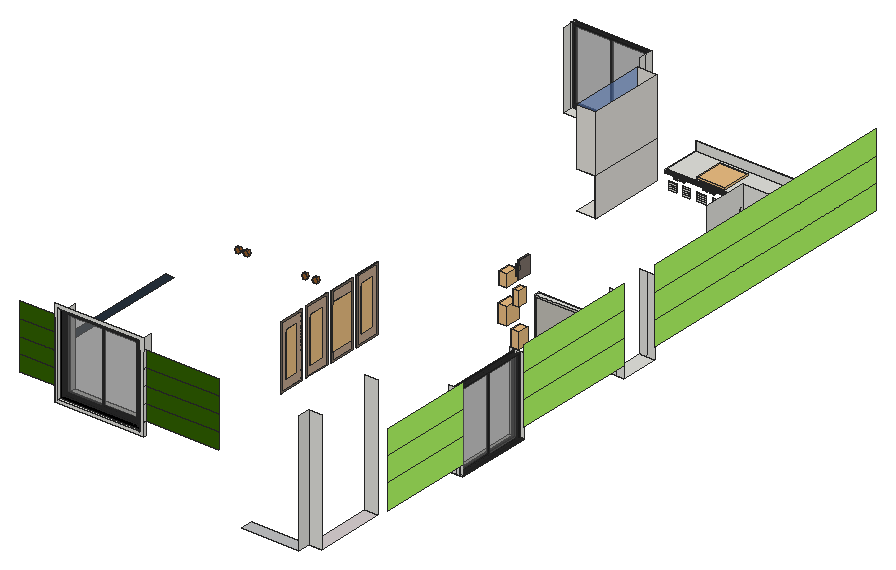
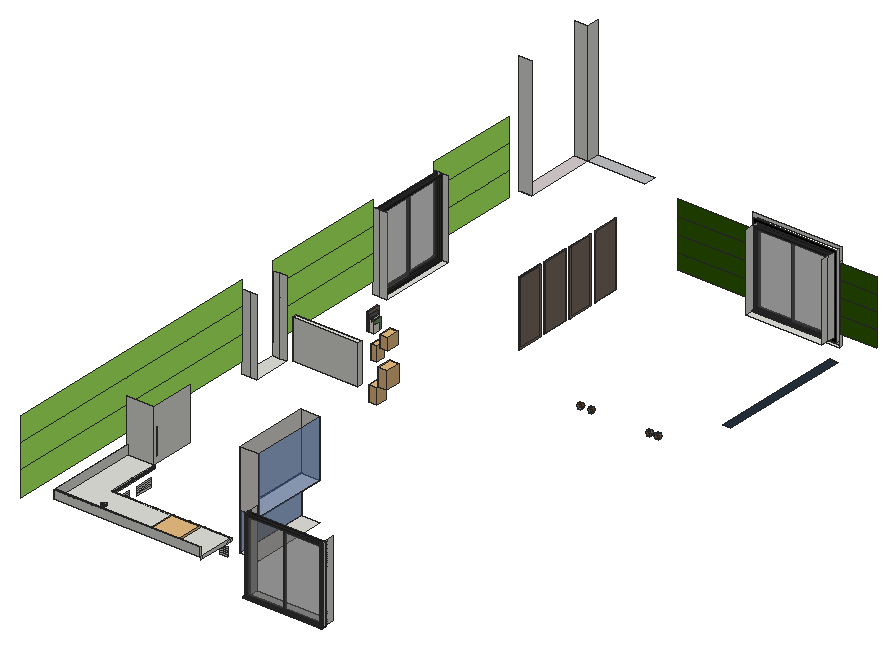
# SketchUp Ruby script. Lengths in inches.
U = 1.inch
M = Sketchup.active_model
def pt(a) = Geom::Point3d.new(a.map { |v| v * U })
def face(e, loops, mat)
  f = e.add_face(loops[0].map { |a| pt(a) })
  loops[1..].each { |l| e.add_face(l.map { |a| pt(a) }).erase! }
  f.material = f.back_material = mat if mat
  f
end
# faces: each face lists its corners as indices into pts; further lists are holes
def faces(e, pts, list, mat = nil) = list.each { |f| face(e, (f[0].is_a?(Array) ? f : [f]).map { |l| l.map { |i| pts[i] } }, mat) }
# xy, xz, yz: faces in a plane at the given z, y or x. An outline is a flat list of corners, or four numbers for a rectangle; further outlines are holes
def ring(l) = l.size == 4 ? [[l[0], l[1]], [l[2], l[1]], [l[2], l[3]], [l[0], l[3]]] : l.each_slice(2).to_a
def flat(e, list, mat, &to3) = list.each { |f| face(e, (f[0].is_a?(Array) ? f : [f]).map { |l| ring(l).map { |u, v| to3.(u, v) } }, mat) }
def xy(e, z, list, mat = nil) = flat(e, list, mat) { |x, y| [x, y, z] }
def xz(e, y, list, mat = nil) = flat(e, list, mat) { |x, z| [x, y, z] }
def yz(e, x, list, mat = nil) = flat(e, list, mat) { |y, z| [x, y, z] }
def lines(e, pts, list) = list.each { |a, b| e.add_line(pt(pts[a]), pt(pts[b])) }
# prism: a flat outline (further loops are holes) pulled along v
def prism(e, loops, v, mat = nil)
  f = face(e, loops, mat); d = Geom::Vector3d.new(v.map { |x| x * U })
  f.pushpull(f.normal.samedirection?(d) ? d.length : -d.length)
end
def box(e, o, s, mat = nil) = prism(e, [[o, [o[0] + s[0], o[1], o[2]], [o[0] + s[0], o[1] + s[1], o[2]], [o[0], o[1] + s[1], o[2]]]], [0, 0, s[2]], mat)
def at(x, y, z, deg = 0) = Geom::Transformation.translation(pt([x, y, z])) * Geom::Transformation.rotation(ORIGIN, Z_AXIS, deg.degrees)
def axes(o, x, y, z) = Geom::Transformation.new([*x, 0, *y, 0, *z, 0, *pt(o).to_a, 1])
def part(name) = M.definitions.add(name)
# library, detail: a bought-in or finely detailed component or shape, given as its bounding box
def library(name, o, s) = part(name).tap { |d| box(d.entities, o, s) }
def detail(e, o, s) = box(e.add_group.entities, o, s)
def put(e, d, t, mat = nil) = e.add_instance(d, t).tap { |i| i.material = mat if mat }
def group(e, t, mat = nil) = e.add_group.tap { |g| g.transformation = t; g.material = mat if mat }.entities
root = M.entities
M.materials.add("[0127_Magenta]").color = [213, 211, 206]
M.materials.add("[0136_Charcoal]").color = [35, 35, 35]
M.materials.add("[1A2796_Cherry-on-Top]1").color = [40, 37, 35]
M.materials.add("[1D2827_Elegant-Rose]").color = [193, 166, 142]
M.materials.add("[1P0222_Buff-Apricot]").color = [122, 108, 96]
M.materials.add("[Color F01]").color = [47, 96, 0]
M.materials.add("[Color F03]").color = [178, 255, 101]
M.materials.add("[Color M09]").color = [0, 0, 0]
M.materials.add("[Color M09]2").color = [194, 192, 183]
M.materials.add("[Color_006]").color = [86, 86, 86]
M.materials.add("[Concrete Pavers Block Multi]").color = [124, 140, 145]
M.materials.add("[Fencing Metal Straight]").color = [194, 195, 196]
M.materials.add("[Fencing Railing Metal]").color = [216, 207, 208]
M.materials.add("[Marble Carrara Gold Floor Tile]").color = [225, 223, 217]
M.materials.add("[Translucent Glass Blue]").color = [100, 149, 237]
M.materials["[Translucent Glass Blue]"].alpha = 0.5
M.materials.add("[Translucent Glass Gray]").color = [117, 117, 117]
M.materials["[Translucent Glass Gray]"].alpha = 0.39
M.materials.add("[Translucent_Glass_Gray]").color = [128, 128, 128]
M.materials["[Translucent_Glass_Gray]"].alpha = 0.5
M.materials.add("[Wood Floor Parquet]").color = [145, 89, 39]
M.materials.add("ksiazki_bialy").color = [255, 246, 235]
M.materials.add("ksiazki_bok").color = [126, 114, 106]
M.materials.add("ksiazki_color").color = [116, 147, 106]
M.materials.add("ksiazki_front").color = [107, 97, 79]
M.materials.add("ksiazki_kolor").color = [96, 96, 96]
M.materials.add("wire_1").color = [39, 49, 60]
c1 = library("Figurine display case",[0,0,0],[10.24,10.24,12.53])
c2 = part("Window")
box(c2.entities,[0,0,0],[39.75,0.5,77],"[Translucent Glass Gray]")
c3 = part("Slider2")
put(c3.entities,c2,at(1.25,1,1.25),"[Translucent Glass Gray]")
c4 = part("Slider")
prism(c4.entities,[[[0,0,0],[42.25,0,0],[42.25,0,79.5],[0,0,79.5]],[[41,0,1.25],[1.25,0,1.25],[1.25,0,78.25],[41,0,78.25]]],[0,1.5,0],"[0136_Charcoal]")
put(c4.entities,c2,at(1.25,1,1.25),"[Translucent_Glass_Gray]")
c5 = part("Frame\#1")
xy(c5.entities,0,[[0,0,88,0.25],[0,6.25,88,6.5]],"[0136_Charcoal]")
xy(c5.entities,1.25,[[-1,6.25,0,9.5],[88,6.25,89,9.5],[0,6.5,88,9.5]],"[0136_Charcoal]")
xy(c5.entities,2,[[2,0.25,86,6.25]],"[0136_Charcoal]")
xy(c5.entities,2.25,[[2.25,0,85.75,1.25],[2.25,2,85.75,5],[2.25,5.75,85.75,6.5],[88,6.25,89,6.25,88,6.5]],"[0136_Charcoal]")
xy(c5.entities,2.75,[[2.75,1.25,85.25,2],[2.75,5,85.25,5.75]],"[0136_Charcoal]")
xy(c5.entities,81.25,[[2.75,1.25,85.25,2],[2.75,5,85.25,5.75]],"[0136_Charcoal]")
xy(c5.entities,81.75,[[2.25,0,85.75,1.25],[2.25,2,85.75,5],[2.25,5.75,85.75,6.5]],"[0136_Charcoal]")
xy(c5.entities,82,[[2,0.25,86,6.25]],"[0136_Charcoal]")
xy(c5.entities,84,[[0,0,88,0.25],[0,6.25,88,6.5]],"[0136_Charcoal]")
xz(c5.entities,0,[[[0,0,88,84],[2.25,2.25,85.75,81.75]]],"[0136_Charcoal]")
xz(c5.entities,0.25,[[[0,0,88,84],[2,2,86,82]]],"[0136_Charcoal]")
xz(c5.entities,1.25,[[[2.25,2.25,85.75,81.75],[2.75,2.75,85.25,81.25]]],"[0136_Charcoal]")
xz(c5.entities,2,[[[2.25,2.25,85.75,81.75],[2.75,2.75,85.25,81.25]]],"[0136_Charcoal]")
xz(c5.entities,5,[[[2.25,2.25,85.75,81.75],[2.75,2.75,85.25,81.25]]],"[0136_Charcoal]")
xz(c5.entities,5.75,[[[2.25,2.25,85.75,81.75],[2.75,2.75,85.25,81.25]]],"[0136_Charcoal]")
xz(c5.entities,6.25,[[[0,0,88,0,88,1.25,89,1.25,89,2.25,88,2.25,88,84,0,84,0,2.25,-1,2.25,-1,1.25,0,1.25],[2,2,86,82]]],"[0136_Charcoal]")
xz(c5.entities,6.5,[[0,0,88,1.25],[0,2.25,0,84,88,84,88,2.25,85.75,2.25,85.75,81.75,2.25,81.75,2.25,2.25]],"[0136_Charcoal]")
xz(c5.entities,9.5,[[-1,1.25,89,1.75]],"[0136_Charcoal]")
yz(c5.entities,-1,[[6.25,1.25,6.25,2.25,9.5,1.75,9.5,1.25]],"[0136_Charcoal]")
yz(c5.entities,0,[[0,0,0.25,84],[6.25,0,6.5,1.25],[6.25,2.25,6.5,84]],"[0136_Charcoal]")
yz(c5.entities,2,[[0.25,2,6.25,82]],"[0136_Charcoal]")
yz(c5.entities,2.25,[[0,2.25,1.25,81.75],[2,2.25,5,81.75],[5.75,2.25,6.5,81.75]],"[0136_Charcoal]")
yz(c5.entities,2.75,[[1.25,2.75,2,81.25],[5,2.75,5.75,81.25]],"[0136_Charcoal]")
yz(c5.entities,85.25,[[1.25,2.75,2,81.25],[5,2.75,5.75,81.25]],"[0136_Charcoal]")
yz(c5.entities,85.75,[[0,2.25,1.25,81.75],[2,2.25,5,81.75],[5.75,2.25,6.5,81.75]],"[0136_Charcoal]")
yz(c5.entities,86,[[0.25,2,6.25,82]],"[0136_Charcoal]")
yz(c5.entities,88,[[0,0,0.25,84],[6.25,0,6.5,1.25],[6.25,2.25,6.5,84]],"[0136_Charcoal]")
yz(c5.entities,89,[[6.25,1.25,9.5,1.25,9.5,1.75,6.25,2.25]],"[0136_Charcoal]")
p = [[89,6.25,2.25],[89,9.5,1.75],[88,6.5,2.25],[-1,6.25,2.25],[0,6.25,2.25],[-1,9.5,1.75],
  [0,6.5,2.25],[2.25,6.5,2.25],[85.75,6.5,2.25]]
faces(c5.entities,p,[[0,1,2],[3,4,5],[6,5,4],[6,7,8,2,1,5]],"[0136_Charcoal]")
put(c5.entities,c3,axes([1.48,-2.48,1.48],[1.01887,0,0],[0,5.47515,0],[0,0,1.01974]))
put(c5.entities,c4,at(43.5,3.5,2.25),"[Color_006]")
c6 = part("Sliding glass door")
put(c6.entities,c5,at(-89,-9.5,-1.25),"[Color_006]")
c7 = library("Range_Countertop\#1",[0,-0.11,0],[27,21.23,1.125])
c8 = library("Figurine display case \#1",[0,0,0],[10.24,10.24,12.53])
c9 = part("faucet_quarter")
xy(c9.entities,0,[[0,0,0,0.97,0.26,0.97,0.71,0.71,0.97,0.26,0.97,0]])
xy(c9.entities,4.5,[[0,0,0.71,0,0.71,0.19,0.52,0.52,0.19,0.71,0,0.71]])
xz(c9.entities,0.97,[[0,0,0.26,4.375]])
yz(c9.entities,0.97,[[0,0,0.26,4.375]])
p = [[0.71,0.71,0],[0.71,0.71,4.375],[0.97,0.26,4.375],[0.97,0.26,0],[0.26,0.97,0],[0.26,0.97,4.375],
  [0.71,0.19,4.5],[0.71,0,4.5],[0.97,0,4.375],[0.52,0.52,4.5],[0.19,0.71,4.5],[0,0.97,4.375],
  [0,0.71,4.5]]
faces(c9.entities,p,[[0,1,2,3],[4,5,1,0],[6,7,8,2],[2,1,9,6],[5,10,9,1],[5,11,12,10]])
c10 = part("Water_Faucet_Sink_Modern")
prism(c10.entities,[[[1.22,-0.07,0.65],[1.02,0.11,0.74],[1.22,0.29,0.83],[1.42,0.11,0.74]]],[0,-0.43,0.9])
xy(c10.entities,2.61,[[-0.12,-2.86,0.11,-0.36]])
xy(c10.entities,3.48,[[-0.11,-3.31,0.12,-0.36]])
xz(c10.entities,-3.31,[[-0.43,3.14,0.44,3.14,0.4375,3.16,0.32,3.36,0.12,3.48,-0.11,3.48,-0.32,3.37,-0.43,3.17]])
xz(c10.entities,-1,[[-0.1875,0.75,0.1875,2.25]])
p = [[-0.01,-3.05,2.56],[0.25,-3.15,2.68],[0.24,-3.34,2.91],[-0.02,-3.43,3.02],[-0.28,-3.33,2.89],[-0.27,-3.14,2.66],
  [-0.12,-2.86,2.61],[0.11,-2.86,2.61],[0.32,-2.96,2.73],[0.43,-3.125,2.93],[0.44,-3.31,3.14],[-0.43,-3.31,3.14],
  [-0.4375,-3.13,2.93],[-0.32,-2.96,2.73],[0.25,-3.01,2.79],[-0.01,-2.91,2.67],[-0.27,-3,2.78],[-0.28,-3.2,3.01],
  [-0.02,-3.3,3.13],[0.24,-3.21,3.02],[-0.12,-0.36,2.61],[-0.32,-0.36,2.73],[0.32,-0.36,2.73],[0.11,-0.36,2.61],
  [-0.4375,-0.36,2.93],[0.43,-0.36,2.93],[-0.43,-3.31,3.17],[-0.43,-0.36,3.17],[0.4375,-3.31,3.16],[0.4375,-0.36,3.16],
  [-0.32,-3.31,3.37],[-0.32,-0.36,3.37],[0.32,-3.31,3.36],[0.32,-0.36,3.36],[-0.11,-3.31,3.48],[-0.11,-0.36,3.48],
  [0.12,-3.31,3.48],[0.12,-0.36,3.48]]
faces(c10.entities,p,[[0,1,2,3,4,5],[[6,7,8,9,10,11,12,13],[14,15,16,17,18,19]],[15,14,1,0],[16,15,0,5],[20,6,13,21],[22,8,7,23],[17,16,5,4],[14,19,2,1],
  [21,13,12,24],[25,9,8,22],[18,17,4,3],[19,18,3,2],[24,12,11,26,27],[28,10,9,25,29],[26,30,31,27],[32,28,29,33],
  [30,34,35,31],[36,32,33,37]])
put(c10.entities,c9,at(0,0,0))
put(c10.entities,c9,at(0,0,0,90))
put(c10.entities,c9,at(0,0,0,180))
put(c10.entities,c9,at(0,0,0,-90))
c11 = part("Group\#8")
xy(c11.entities,0,[[[-2.25,-2.38,53.86,142.58],[0,0,51.61,140.2]],[0,0,51.61,140.2]])
xy(c11.entities,0.7,[[[-2.25,-2.38,53.86,142.58],[0,0,51.61,140.2]]])
xy(c11.entities,0.7,[[0,0,51.61,140.2]],"[1D2827_Elegant-Rose]")
xy(c11.entities,1.41,[[[-2.25,-2.38,53.86,142.58],[0,0,51.61,140.2]]],"[1P0222_Buff-Apricot]")
xz(c11.entities,-2.38,[[-2.25,0,53.86,0.7],[-2.25,0.7,53.86,1.41]])
xz(c11.entities,0,[[0,0,51.61,0.7],[0,0.7,51.61,1.41]])
xz(c11.entities,140.2,[[0,0,51.61,0.7],[0,0.7,51.61,1.41]])
xz(c11.entities,142.58,[[-2.25,0,53.86,0.7],[-2.25,0.7,53.86,1.41]])
yz(c11.entities,-2.25,[[-2.38,0,142.58,0.7],[-2.38,0.7,142.58,1.41]])
yz(c11.entities,0,[[0,0,140.2,0.7],[0,0.7,140.2,1.41]])
yz(c11.entities,51.61,[[0,0,140.2,0.7],[0,0.7,140.2,1.41]])
yz(c11.entities,53.86,[[-2.38,0,142.58,0.7],[-2.38,0.7,142.58,1.41]])
c12 = library("Group\#17",[0,0,0],[49.77,99.98,0.7])
c13 = library("Groupe\#36",[0,0,0],[8.85,8.01,13.18])
c14 = library("Group\#7",[0,0,0],[32.82,100.33,0.7])
c15 = library("Group\#10",[0,0,0],[29.16,100.07,0.7])
c16 = library("Group\#6",[0,0,0],[27.2,98.94,0.7])
c17 = library("vase3mm",[-1.8,-1.8,0],[3.6,3.6,4.77])
c18 = part("books")
g1 = group(c18.entities,at(0,-187.6875,-13.27))
xy(g1,13.89,[[0,1.25,0,67.05,71.57,67.05,71.57,5.87,43.27,5.87,43.27,1.25],[0,68.28,98.43,86.07]],"ksiazki_front")
xy(g1,69.43,[[0,0,43.27,5.87]],"ksiazki_bialy")
xy(g1,89.27,[[0,21.18,71.57,31.42]],"ksiazki_bialy")
xy(g1,90.86,[[0,5.87,71.57,19.73]],"ksiazki_bialy")
xy(g1,91.92,[[0,19.73,71.57,21.18]],"ksiazki_bialy")
xy(g1,101.14,[[0,31.42,71.57,40.16]],"ksiazki_bialy")
xy(g1,105.94,[[0,40.16,71.57,48.94]],"ksiazki_bialy")
xy(g1,124.42,[[0,57.01,71.57,67.05]],"ksiazki_bialy")
xy(g1,127.59,[[0,48.94,71.57,57.01]],"ksiazki_bialy")
xz(g1,5.87,[[43.27,13.89,71.57,13.89,71.57,90.86,0,90.86,0,69.43,43.27,69.43]],"ksiazki_color")
xz(g1,19.73,[[0,90.86,71.57,91.92]],"ksiazki_front")
xz(g1,21.18,[[0,89.27,71.57,91.92]],"ksiazki_front")
xz(g1,31.42,[[0,89.27,71.57,101.14]],"ksiazki_bialy")
xz(g1,40.16,[[0,101.14,71.57,105.94]],"ksiazki_color")
xz(g1,48.94,[[0,105.94,71.57,127.59]],"ksiazki_kolor")
xz(g1,57.01,[[0,124.42,71.57,127.59]],"ksiazki_front")
xz(g1,67.05,[[0,13.89,71.57,124.42]],"ksiazki_front")
yz(g1,0,[[1.25,13.89,0,69.43,5.87,69.43,5.87,90.86,19.73,90.86,19.73,91.92,21.18,91.92,21.18,89.27,31.42,89.27,31.42,101.14,40.16,101.14,40.16,105.94,48.94,105.94,48.94,127.59,57.01,127.59,57.01,124.42,67.05,124.42,67.05,13.89],[68.28,13.89,69.91,143.31,89.63,141.875,86.07,13.89]],"ksiazki_bialy")
yz(g1,43.27,[[1.25,13.89,5.87,13.89,5.87,69.43,0,69.43]],"ksiazki_front")
yz(g1,71.57,[[5.87,13.89,67.05,13.89,67.05,124.42,57.01,124.42,57.01,127.59,48.94,127.59,48.94,105.94,40.16,105.94,40.16,101.14,31.42,101.14,31.42,89.27,21.18,89.27,21.18,91.92,19.73,91.92,19.73,90.86,5.87,90.86]],"ksiazki_front")
yz(g1,98.43,[[68.28,13.89,86.07,13.89,89.63,141.875,69.91,143.31]],"ksiazki_front")
p = [[0,0,69.43],[0,1.25,13.89],[43.27,1.25,13.89],[43.27,0,69.43],[98.43,68.28,13.89],[98.43,69.91,143.31],
  [0,69.91,143.31],[0,68.28,13.89],[0,86.07,13.89],[0,89.63,141.875],[98.43,89.63,141.875],[98.43,86.07,13.89]]
faces(g1,p,[[0,1,2,3]])
faces(g1,p,[[4,5,6,7],[8,9,10,11]],"ksiazki_bok")
faces(g1,p,[[9,6,5,10]],"ksiazki_bialy")
xy(root,70.43,[[32.01,58,88.01,60]])
xy(root,72.43,[[34.01,58,86.01,60]])
xy(root,74.1,[[175.27,411.4,178.125,411.72]])
xy(root,74.43,[[36.01,60,84.01,69],[231,118.97,240,166.97],[231,245.63,240,269.63],[50.67,435,98.67,444]])
xy(root,74.43,[[117,361.98,128.3125,409.98],[128.3125,361.98,129,409.98]],"[Marble Carrara Gold Floor Tile]")
xy(root,74.65,[[175.27,411.4,178.125,411.72]])
xy(root,77.72,[[184.47,245.35,225.41,248.23]])
xy(root,78.19,[[196.33,411.4,199.18,411.72]])
xy(root,78.41,[[161.46,411.4,164.3125,411.72]])
xy(root,78.52,[[142.6,411.4,145.45,411.72],[191.81,411.4,194.66,411.72]])
xy(root,78.54,[[157.16,411.4,160.01,411.72]])
xy(root,78.57,[[138.5625,411.4,141.42,411.72]])
xy(root,78.74,[[196.33,411.4,199.18,411.72]])
xy(root,78.96,[[161.46,411.4,164.3125,411.72]])
xy(root,79.06,[[191.81,411.4,194.66,411.72]])
xy(root,79.07,[[142.6,411.4,145.45,411.72]])
xy(root,79.08,[[157.16,411.4,160.01,411.72]])
xy(root,79.12,[[138.5625,411.4,141.42,411.72]])
xy(root,82.07,[[208.39,378.03,208.39,411.72,133.5,411.72,133.5,435.01,225.1,435.01,225.1,378.03]])
xy(root,82.43,[[196,0,232,8]],"[Fencing Metal Straight]")
xy(root,82.43,[[232,8,240,52]],"[Fencing Railing Metal]")
xy(root,83.36,[[9,90.07,14.125,174.1]],"wire_1")
xy(root,87.52,[[225.1,378.03,225.1,435.01,133.5,435.01,133.5,435.8125,225.68,435.8125,225.68,378.03]])
xy(root,98.43,[[117,361.98,128.3125,409.98],[128.3125,361.98,129,409.98]],"[Marble Carrara Gold Floor Tile]")
xy(root,102.28,[[184.47,245.35,225.41,248.23]])
xz(root,8,[[232,82.43,240,158.43]])
xz(root,52,[[232,82.43,240,158.43]])
xz(root,58,[[[32.01,70.43,88.01,126.43],[34.01,72.43,86.01,124.43]]])
xz(root,60,[[9,78.43,32.01,88.43],[88.01,78.43,133.5,88.43],[9,88.43,32.01,98.43],[88.01,88.43,133.5,98.43],[9,98.43,32.01,108.43],
  [88.01,98.43,133.5,108.43],[9,108.43,32.01,118.43],[88.01,108.43,133.5,118.43]],"[Color F01]")
xz(root,60,[[[34.01,72.43,86.01,124.43],[36.01,74.43,84.01,122.43]]],"[Color M09]")
xz(root,118.97,[[231,74.43,235.5,123.43],[235.5,74.43,240,123.43]])
xz(root,166.97,[[231,74.43,235.5,123.43],[235.5,74.43,240,123.43]])
xz(root,208.5,[[74.6,86.41,76.49,86.43,77.41,88.07,76.45,89.69,74.5625,89.67,73.64,88.03],[25.97,86.42,27.81,86.43,28.72,88.03,27.8,89.62,25.96,89.61,25.04,88.02],[33.0625,86.43,33.99,88,33.1,89.59,31.28,89.61,30.35,88.05,31.24,86.45],[69.76,86.43,70.7,88.03,69.79,89.65,67.93,89.67,66.98,88.07,67.9,86.45]],"[Wood Floor Parquet]")
xz(root,245.35,[[[184.47,77.72,225.41,102.28],[185.68,78.93,224.2,101.08]],[185.68,78.93,224.2,101.08]],"[Color M09]2")
xz(root,245.63,[[231,74.43,235.5,122.43],[235.5,74.43,240,122.43]])
xz(root,248.23,[[184.47,77.72,225.41,102.28]])
xz(root,269.63,[[231,74.43,235.5,122.43],[235.5,74.43,240,122.43]])
xz(root,361.98,[[128.3125,74.43,129,98.43],[117,98.43,129,134.43]],"[Marble Carrara Gold Floor Tile]")
xz(root,378.03,[[208.39,79.89,208.27,79.98,208.17,80.12,208.08,80.29,208.02,80.5,207.98,80.73,207.96,80.98,207.98,81.22,208.02,81.45,208.08,81.66,208.17,81.84,208.27,81.97,208.39,82.07],[208.97,82.07,225.1,82.07,225.1,87.52,225.68,87.52,225.68,114.79,208.97,114.79]])
xz(root,409.98,[[128.3125,74.43,129,98.43],[117,98.43,129,134.43]],"[Marble Carrara Gold Floor Tile]")
xz(root,411.4,[[175.27,74.1,178.125,74.65],[196.33,78.19,199.18,78.74],[161.46,78.41,164.3125,78.96],[142.6,78.52,145.45,79.07],[191.81,78.52,194.66,79.06],
  [157.16,78.54,160.01,79.08],[138.5625,78.57,141.42,79.12]])
xz(root,411.72,[[144.16,70.61,148.77,71.7],[162.88,70.61,168.93,71.7],[[171.8125,70.61,181.6,78.25],[172.1,71.16,181.32,77.7]],[184.49,70.61,193.41,71.7],[197.45,70.61,206.38,71.7],
  [152.8,70.91,158.85,72],[135.52,70.95,140.125,72.04],[[172.1,71.16,181.32,77.7],[175.27,74.1,178.125,74.65]],[144.16,71.7,148.77,72.79],[162.88,71.7,168.93,72.79],
  [184.49,71.7,193.41,72.79],[197.45,71.7,206.38,72.79],[152.8,72,158.85,73.1],[135.52,72.04,140.125,73.13],[144.16,72.79,148.77,73.89],
  [162.88,72.79,168.93,73.89],[184.49,72.79,193.41,73.89],[197.45,72.79,206.38,73.89],[152.8,73.1,158.85,74.1875],[135.52,73.13,140.125,74.22],
  [144.16,73.89,148.77,74.98],[162.88,73.89,168.93,74.98],[184.49,73.89,193.41,74.98],[197.45,73.89,206.38,74.98],[152.8,74.1875,158.85,75.28],
  [135.52,74.22,140.125,75.3125],[144.16,74.98,148.77,76.07],[162.88,74.98,168.93,76.07],[184.49,74.98,193.41,76.07],[197.45,74.98,206.38,76.07],
  [152.8,75.28,158.85,76.07],[135.52,75.3125,140.125,76.07],[133.5,79.89,170.95,82.07],[170.95,79.89,182.47,82.07],[182.47,79.89,208.39,82.07]])
xz(root,435.01,[[133.5,82.07,225.1,87.52]])
xz(root,435.8125,[[133.5,82.07,225.68,87.52]])
yz(root,32.01,[[58,70.43,60,78.43],[58,78.43,60,88.43],[58,88.43,60,98.43],[58,98.43,60,108.43],[58,108.43,60,118.43]])
yz(root,34.01,[[58,72.43,60,124.43]])
yz(root,36.01,[[60,74.43,64.09,122.43],[64.09,74.43,69,122.43]])
yz(root,50.67,[[435,74.43,439.5,122.43],[439.5,74.43,444,122.43]])
yz(root,84.01,[[60,74.43,69,122.43]])
yz(root,86.01,[[58,72.43,60,88.43],[58,88.43,60,98.43],[58,98.43,60,108.43],[58,108.43,60,118.43]])
yz(root,88.01,[[58,70.43,60,78.43],[58,78.43,60,88.43],[58,88.43,60,98.43],[58,98.43,60,108.43],[58,108.43,60,118.43]])
yz(root,98.67,[[435,74.43,439.5,122.43],[439.5,74.43,444,122.43]])
yz(root,117,[[361.98,98.43,409.98,134.43]],"[Translucent Glass Blue]")
yz(root,128.3125,[[361.98,74.43,409.98,98.43]],"[Translucent Glass Blue]")
yz(root,129,[[361.98,74.43,409.98,98.43],[361.98,98.43,409.98,134.43]],"[Marble Carrara Gold Floor Tile]")
yz(root,133.5,[[411.72,79.89,411.72,82.07,411.55,81.97,411.41,81.84,411.28,81.66,411.19,81.45,411.14,81.22,411.12,80.98,411.14,80.73,411.19,80.5,411.28,80.29,411.41,80.12,411.55,79.98],[411.72,79.89,415.76,79.89,411.72,82.07],[415.76,79.89,434.1875,79.89,434.1875,82.07,411.72,82.07],[434.1875,79.89,435.01,82.07],[435.01,82.07,435.8125,87.52]])
yz(root,138.5625,[[411.4,78.57,411.72,79.12]])
yz(root,141.42,[[411.4,78.57,411.72,79.12]])
yz(root,142.6,[[411.4,78.52,411.72,79.07]])
yz(root,145.45,[[411.4,78.52,411.72,79.07]])
yz(root,157.16,[[411.4,78.54,411.72,79.08]])
yz(root,160.01,[[411.4,78.54,411.72,79.08]])
yz(root,161.46,[[411.4,78.41,411.72,78.96]])
yz(root,164.3125,[[411.4,78.41,411.72,78.96]])
yz(root,175.27,[[411.4,74.1,411.72,74.65]])
yz(root,178.125,[[411.4,74.1,411.72,74.65]])
yz(root,184.47,[[245.35,77.72,248.23,102.28]])
yz(root,191.81,[[411.4,78.52,411.72,79.06]])
yz(root,194.66,[[411.4,78.52,411.72,79.06]])
yz(root,196.33,[[411.4,78.19,411.72,78.74]])
yz(root,199.18,[[411.4,78.19,411.72,78.74]])
yz(root,208.39,[[381.11,70.61,392.0625,71.7],[397.95,70.61,408.91,71.7],[381.11,71.7,392.0625,72.79],[397.95,71.7,408.91,72.79],[381.11,72.79,392.0625,73.89],
  [397.95,72.79,408.91,73.89],[381.11,73.89,392.0625,74.98],[397.95,73.89,408.91,74.98],[381.11,74.98,392.0625,76.07],[397.95,74.98,408.91,76.07]])
yz(root,208.97,[[[349.92,82.07,378.03,114.79],[374.49,85.54,376.18,102.45]],[374.49,85.54,376.18,102.45]])
yz(root,225.1,[[378.03,82.07,435.01,87.52]])
yz(root,225.41,[[245.35,77.72,248.23,102.28]])
yz(root,225.68,[[378.03,82.07,435.8125,87.52]])
yz(root,232,[[0,82.43,8,158.43]])
yz(root,240,[[60,81.56,118.97,96.93],[166.97,81.56,245.63,96.93],[269.63,81.56,444,96.93],[60,96.93,118.97,112.31],[166.97,96.93,245.63,112.31],
  [269.63,96.93,444,112.31],[60,112.31,118.97,127.68],[166.97,112.31,245.63,127.68],[269.63,112.31,444,127.68]],"[Color F03]")
p = [[208.39,411.72,79.89],[208.27,411.55,79.98],[208.27,394.875,79.98],[208.27,378.03,79.98],[208.39,378.03,79.89],[208.39,394.875,79.89],
  [195.43,411.55,79.98],[195.43,411.72,79.89],[182.47,411.72,79.89],[170.95,411.72,79.89],[160.86,411.72,79.89],[150.78,411.72,79.89],
  [142.14,411.72,79.89],[133.5,411.72,79.89],[133.5,411.55,79.98],[142.14,411.55,79.98],[150.78,411.55,79.98],[160.86,411.55,79.98],
  [170.95,411.55,79.98],[182.47,411.55,79.98],[208.17,394.875,80.12],[208.17,378.03,80.12],[208.17,411.41,80.12],[150.78,411.41,80.12],
  [160.86,411.41,80.12],[170.95,411.41,80.12],[182.47,411.41,80.12],[195.43,411.41,80.12],[133.5,411.41,80.12],[142.14,411.41,80.12],
  [208.08,394.875,80.29],[208.08,378.03,80.29],[208.08,411.28,80.29],[150.78,411.28,80.29],[160.86,411.28,80.29],[170.95,411.28,80.29],
  [182.47,411.28,80.29],[195.43,411.28,80.29],[133.5,411.28,80.29],[142.14,411.28,80.29],[208.02,411.19,80.5],[208.02,394.875,80.5],
  [208.02,378.03,80.5],[150.78,411.19,80.5],[160.86,411.19,80.5],[170.95,411.19,80.5],[182.47,411.19,80.5],[195.43,411.19,80.5],
  [133.5,411.19,80.5],[142.14,411.19,80.5],[207.98,411.14,80.73],[207.98,394.875,80.73],[207.98,378.03,80.73],[150.78,411.14,80.73],
  [160.86,411.14,80.73],[170.95,411.14,80.73],[182.47,411.14,80.73],[195.43,411.14,80.73],[133.5,411.14,80.73],[142.14,411.14,80.73],
  [207.96,411.12,80.98],[207.96,394.875,80.98],[207.96,378.03,80.98],[150.78,411.12,80.98],[160.86,411.12,80.98],[170.95,411.12,80.98],
  [182.47,411.12,80.98],[195.43,411.12,80.98],[133.5,411.12,80.98],[142.14,411.12,80.98],[207.98,411.14,81.22],[207.98,394.875,81.22],
  [207.98,378.03,81.22],[150.78,411.14,81.22],[160.86,411.14,81.22],[170.95,411.14,81.22],[182.47,411.14,81.22],[195.43,411.14,81.22],
  [133.5,411.14,81.22],[142.14,411.14,81.22],[208.02,411.19,81.45],[208.02,394.875,81.45],[208.02,378.03,81.45],[150.78,411.19,81.45],
  [160.86,411.19,81.45],[170.95,411.19,81.45],[182.47,411.19,81.45],[195.43,411.19,81.45],[133.5,411.19,81.45],[142.14,411.19,81.45],
  [208.08,411.28,81.66],[208.08,394.875,81.66],[208.08,378.03,81.66],[195.43,411.28,81.66],[133.5,411.28,81.66],[142.14,411.28,81.66],
  [150.78,411.28,81.66],[160.86,411.28,81.66],[170.95,411.28,81.66],[182.47,411.28,81.66],[208.17,411.41,81.84],[208.17,394.875,81.84],
  [208.17,378.03,81.84],[195.43,411.41,81.84],[133.5,411.41,81.84],[142.14,411.41,81.84],[150.78,411.41,81.84],[160.86,411.41,81.84],
  [170.95,411.41,81.84],[182.47,411.41,81.84],[208.27,411.55,81.97],[208.27,394.875,81.97],[208.27,378.03,81.97],[195.43,411.55,81.97],
  [133.5,411.55,81.97],[142.14,411.55,81.97],[150.78,411.55,81.97],[160.86,411.55,81.97],[170.95,411.55,81.97],[182.47,411.55,81.97],
  [208.39,411.72,82.07],[208.39,394.875,82.07],[208.39,378.03,82.07],[195.43,411.72,82.07],[133.5,411.72,82.07],[142.14,411.72,82.07],
  [150.78,411.72,82.07],[160.86,411.72,82.07],[170.95,411.72,82.07],[182.47,411.72,82.07],[25.04,210,88.02],[25.97,210,86.42],
  [25.97,208.5,86.42],[25.04,208.5,88.02],[27.81,210,86.43],[27.81,208.5,86.43],[28.72,210,88.03],[28.72,208.5,88.03],
  [31.24,210,86.45],[33.0625,210,86.43],[33.0625,208.5,86.43],[31.24,208.5,86.45],[33.99,210,88],[33.99,208.5,88],
  [66.98,210,88.07],[67.9,210,86.45],[67.9,208.5,86.45],[66.98,208.5,88.07],[69.76,210,86.43],[69.76,208.5,86.43],
  [70.7,210,88.03],[70.7,208.5,88.03],[73.64,210,88.03],[74.6,210,86.41],[74.6,208.5,86.41],[73.64,208.5,88.03],
  [76.49,210,86.43],[76.49,208.5,86.43],[77.41,210,88.07],[77.41,208.5,88.07],[30.35,210,88.05],[30.35,208.5,88.05],
  [25.96,210,89.61],[25.96,208.5,89.61],[27.8,210,89.62],[27.8,208.5,89.62],[31.28,210,89.61],[31.28,208.5,89.61],
  [33.1,210,89.59],[33.1,208.5,89.59],[69.79,210,89.65],[69.79,208.5,89.65],[74.5625,210,89.67],[74.5625,208.5,89.67],
  [67.93,210,89.67],[67.93,208.5,89.67],[76.45,210,89.69],[76.45,208.5,89.69]]
faces(root,p,[[0,1,2,3,4,5],[6,1,0,7,8,9,10,11,12,13,14,15,16,17,18,19],[20,21,3,2,1,22],[23,24,25,26,27,22,1,6,19,18,17,16,15,14,28,29],[30,31,21,20,22,32],[33,34,35,36,37,32,22,27,26,25,24,23,29,28,38,39],[32,40,41,42,31,30],[43,44,45,46,47,40,32,37,36,35,34,33,39,38,48,49],
  [40,50,51,52,42,41],[53,54,55,56,57,50,40,47,46,45,44,43,49,48,58,59],[50,60,61,62,52,51],[63,64,65,66,67,60,50,57,56,55,54,53,59,58,68,69],[60,70,71,72,62,61],[73,74,75,76,77,70,60,67,66,65,64,63,69,68,78,79],[70,80,81,82,72,71],[83,84,85,86,87,80,70,77,76,75,74,73,79,78,88,89],
  [80,90,91,92,82,81],[93,90,80,87,86,85,84,83,89,88,94,95,96,97,98,99],[90,100,101,102,92,91],[103,100,90,93,99,98,97,96,95,94,104,105,106,107,108,109],[100,110,111,112,102,101],[113,110,100,103,109,108,107,106,105,104,114,115,116,117,118,119],[110,120,121,122,112,111],[123,120,110,113,119,118,117,116,115,114,124,125,126,127,128,129]])
faces(root,p,[[130,131,132,133],[131,134,135,132],[138,139,140,141],[145,148,149,146],[148,150,151,149],[153,156,157,154],[156,158,159,157],[160,138,141,161],
  [162,130,133,163],[166,160,161,167]],"[Concrete Pavers Block Multi]")
faces(root,p,[[134,136,137,135],[139,142,143,140],[144,145,146,147],[152,153,154,155],[136,164,165,137],[142,168,169,143],[150,170,171,151],[172,152,155,173],
  [174,144,147,175],[158,176,177,159],[164,162,163,165],[168,166,167,169],[170,174,175,171],[176,172,173,177]],"[Wood Floor Parquet]")
put(root,c1,axes([173.0625,240.7,70.95],[0.48625,0,0],[0,0.6978,0],[0,0,0.79]))
put(root,c6,axes([240,118.97,74.9],[0,-0.52733,0],[0.60109,0,0],[0,0,0.58644]),"[0127_Magenta]")
put(root,c6,axes([84.01,64.61,75.15],[0.53333,0,0],[0,0.48475,0],[0,0,0.57143]),"[0127_Magenta]")
put(root,c6,axes([49.39,445.12,75.15],[-0.5537,0,0],[0,0.37268,0],[0,0,0.57143]),"[0127_Magenta]")
put(root,c7,axes([151.69,413.6,82.07],[0.65117,0,0],[0,0.83966,0],[0,0,0.97665]))
put(root,c8,axes([165.67,239.63,82.41],[0.54164,0,0],[0,0.88,0],[0,0,0.88]))
put(root,c10,axes([197.17,433.16,82.41],[0.73165,0,0],[0,1.02,0],[0,0,1.38545]))
put(root,c11,axes([133.5,124.82,89.24],[0,-0.2968,0],[0,0,0.28],[0.28,0,0]),"[1P0222_Buff-Apricot]")
put(root,c11,axes([133.5,144.625,89.24],[0,-0.2968,0],[0,0,0.28],[0.28,0,0]),"[1P0222_Buff-Apricot]")
put(root,c11,axes([133.5,184.23,89.24],[0,-0.2968,0],[0,0,0.28],[0.28,0,0]),"[1P0222_Buff-Apricot]")
put(root,c11,axes([133.5,164.43,89.24],[0,-0.2968,0],[0,0,0.28],[0.28,0,0]),"[1P0222_Buff-Apricot]")
put(root,c12,axes([133.7,163.71,94.03],[0,-0.28,0],[0,0,0.28],[0.28,0,0]),"[1A2796_Cherry-on-Top]1")
put(root,c13,axes([177.51,246.72,94.57],[-0.41239,0,0],[0,-0.67,0],[0,0,0.67]))
put(root,c14,axes([133.7,141.22,94.76],[0,-0.28,0],[0,0,0.28],[0.28,0,0]),"[1A2796_Cherry-on-Top]1")
put(root,c15,axes([133.7,180.22,94.82],[0,-0.28,0],[0,0,0.28],[0.28,0,0]),"[1A2796_Cherry-on-Top]1")
put(root,c16,axes([133.7,120.74,95.08],[0,-0.28,0],[0,0,0.28],[0.28,0,0]),"[1A2796_Cherry-on-Top]1")
put(root,c17,axes([168.52,243.75,104.01],[0,2.2743,0],[-1.39984,0,0],[0,0,1.56927]))
g2 = group(root,at(167.46,239.81,110.74))
put(g2,c18,axes([16.3,8.23,0.15],[0,-0.0836,0],[0.0493,0,0],[0,0,0.0836]))
